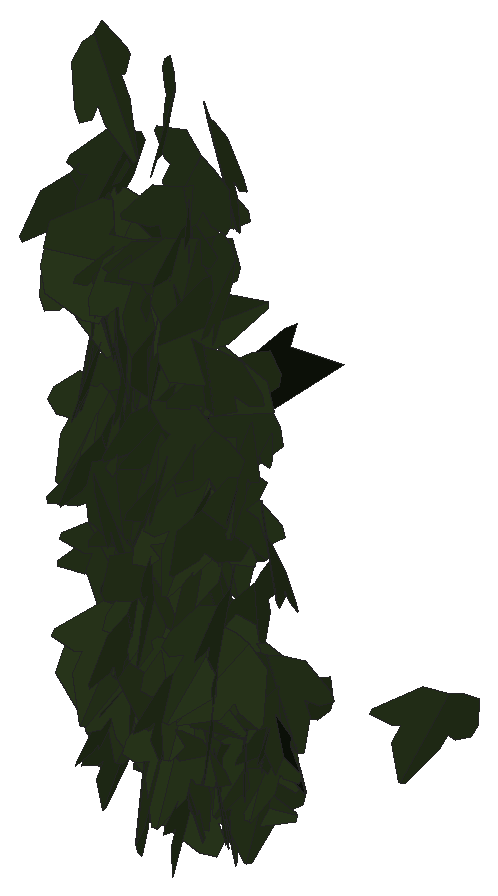
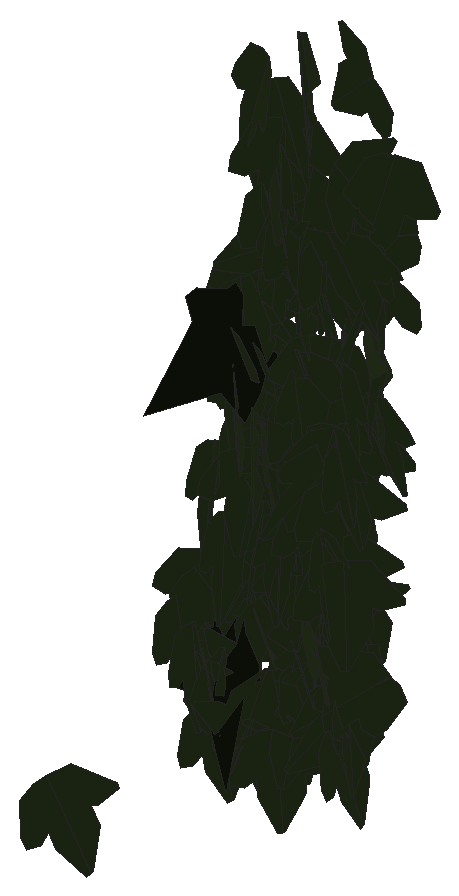
# SketchUp Ruby script. Lengths in inches.
U = 1.inch
M = Sketchup.active_model
def pt(a) = Geom::Point3d.new(a.map { |v| v * U })
def face(e, loops, mat)
  f = e.add_face(loops[0].map { |a| pt(a) })
  loops[1..].each { |l| e.add_face(l.map { |a| pt(a) }).erase! }
  f.material = f.back_material = mat if mat
  f
end
# faces: each face lists its corners as indices into pts; further lists are holes
def faces(e, pts, list, mat = nil) = list.each { |f| face(e, (f[0].is_a?(Array) ? f : [f]).map { |l| l.map { |i| pts[i] } }, mat) }
# xy, xz, yz: faces in a plane at the given z, y or x. An outline is a flat list of corners, or four numbers for a rectangle; further outlines are holes
def ring(l) = l.size == 4 ? [[l[0], l[1]], [l[2], l[1]], [l[2], l[3]], [l[0], l[3]]] : l.each_slice(2).to_a
def flat(e, list, mat, &to3) = list.each { |f| face(e, (f[0].is_a?(Array) ? f : [f]).map { |l| ring(l).map { |u, v| to3.(u, v) } }, mat) }
def xy(e, z, list, mat = nil) = flat(e, list, mat) { |x, y| [x, y, z] }
def xz(e, y, list, mat = nil) = flat(e, list, mat) { |x, z| [x, y, z] }
def yz(e, x, list, mat = nil) = flat(e, list, mat) { |y, z| [x, y, z] }
def lines(e, pts, list) = list.each { |a, b| e.add_line(pt(pts[a]), pt(pts[b])) }
# prism: a flat outline (further loops are holes) pulled along v
def prism(e, loops, v, mat = nil)
  f = face(e, loops, mat); d = Geom::Vector3d.new(v.map { |x| x * U })
  f.pushpull(f.normal.samedirection?(d) ? d.length : -d.length)
end
def box(e, o, s, mat = nil) = prism(e, [[o, [o[0] + s[0], o[1], o[2]], [o[0] + s[0], o[1] + s[1], o[2]], [o[0], o[1] + s[1], o[2]]]], [0, 0, s[2]], mat)
def at(x, y, z, deg = 0) = Geom::Transformation.translation(pt([x, y, z])) * Geom::Transformation.rotation(ORIGIN, Z_AXIS, deg.degrees)
def axes(o, x, y, z) = Geom::Transformation.new([*x, 0, *y, 0, *z, 0, *pt(o).to_a, 1])
def part(name) = M.definitions.add(name)
# library, detail: a bought-in or finely detailed component or shape, given as its bounding box
def library(name, o, s) = part(name).tap { |d| box(d.entities, o, s) }
def detail(e, o, s) = box(e.add_group.entities, o, s)
def put(e, d, t, mat = nil) = e.add_instance(d, t).tap { |i| i.material = mat if mat }
def group(e, t, mat = nil) = e.add_group.tap { |g| g.transformation = t; g.material = mat if mat }.entities
root = M.entities
M.materials.add("efeu1").color = [18, 25, 13]
M.materials.add("efeu2").color = [43, 57, 29]
c1 = part("ivyleaf_10")
p = [[0,0.5,-0.03],[-0.0625,2.02,-0.43],[-0.19,2.01,-0.46],[-0.54,1.05,-0.29],[-0.52,0.625,-0.18],[-0.83,0.76,-0.28],
  [-1.16,0.64,-0.33],[-1.15,0.33,-0.24],[-0.77,-0.39,0.02],[-0.3,-0.51,0.16],[0.04,-0.48,0.23],[-0.02,2.01,-0.4375],
  [-0.06,2.01,-0.43],[0.04,-0.49,0.23],[0.67,-0.49,0.14],[1.38,0.36,-0.2],[1.375,0.51,-0.24],[0.81,0.65,-0.19],
  [0.62,0.59,-0.15],[0.6,1.09,-0.28],[0.5,1.23,-0.31]]
faces(c1.entities,p,[[0,1,2,3,4,5,6,7,8,9,10],[11,12,0,13,14,15,16,17,18,19,20]],"efeu2")
c2 = part("ivyleaf_9")
p = [[1.54,2.16,1.25],[1.36,2.04,1.19],[-0.21,0.99,0.68],[-0.71,1.11,0.82],[-0.85,0.86,0.67],[-0.8,0.17,0.21],
  [-0.9,-0.01,0.1],[-0.67,-0.16,-0.02],[-0.08,-0.08,-0.05],[-0.03,-0.6,-0.4],[0.65,-0.88,-0.66],[0.83,-0.6,-0.49],
  [1.29,-0.42,-0.43],[1.8125,-0.07,-0.26],[1.21,0.44,0.15]]
faces(c2.entities,p,[[0,1,2,3,4,5,6,7,8,9,10,11,12,13,14]],"efeu1")
put(root,c1,axes([518.78,137.96,175.26],[-0.50751,-0.42588,0.04296],[-0.02362,-0.03868,-0.66237],[0.42739,-0.50785,0.01442]))
put(root,c1,axes([518.52,137.62,178.78],[-0.20052,0.24162,-0.60735],[0.13881,-0.60506,-0.28654],[-0.63874,-0.20734,0.1284]))
put(root,c1,axes([518.83,137.2,178.78],[0.29577,-0.57193,-0.26548],[-0.1065,0.24371,-0.64368],[0.62148,0.31395,0.01603]))
put(root,c1,axes([518.79,138.03,172.45],[0.05616,-0.64726,0.09818],[-0.00689,-0.09912,-0.64952],[0.65463,0.05449,-0.01526]))
put(root,c1,axes([518.35,137.83,173.59],[0.30727,0.26062,0.59411],[0.37634,0.46386,-0.39812],[-0.52845,0.48189,0.06192]))
put(root,c1,axes([518.9375,137.88,175.5625],[-0.4811,-0.41426,0.20769],[-0.13167,-0.16484,-0.6338],[0.44431,-0.49741,0.03707]))
put(root,c1,axes([518.85,137.18,177.88],[0.61337,-0.23963,-0.19798],[-0.18385,0.07347,-0.65852],[0.25064,0.64033,0.00147]))
put(root,c1,axes([518.9,137.61,173.06],[0.08241,-0.64908,-0.2337],[-0.04843,0.22934,-0.65404],[0.68817,0.09387,-0.01805]))
put(root,c1,axes([518.91,137.01,180.29],[0.45498,-0.40858,-0.34243],[-0.13516,0.34708,-0.59369],[0.51568,0.45145,0.14652]))
put(root,c1,axes([518.89,137.69,177.22],[-0.03414,-0.68527,0.01798],[0.00158,-0.01808,-0.68611],[0.6855,-0.03408,0.00247]))
put(root,c1,axes([519.05,137.875,177.49],[-0.61947,0.2017,0.17565],[-0.22489,-0.15298,-0.61749],[-0.14476,-0.62545,0.20768]))
put(root,c1,axes([518.98,137.75,176.5625],[-0.45983,-0.47966,0.11029],[-0.00425,-0.14707,-0.6573],[0.49216,-0.44942,0.09737]))
put(root,c1,axes([518.89,136.72,181.65],[-0.2605,-0.60194,-0.31695],[0.1428,0.28344,-0.65568],[0.66513,-0.29661,0.01664]))
put(root,c1,axes([518.54,137.18,180.16],[0.54281,0.04361,0.4176],[0.41722,0.02047,-0.54446],[-0.04706,0.68455,-0.01032]))
put(root,c1,axes([518.84,137.7,173.01],[-0.11754,-0.29919,-0.63473],[0.22771,0.59248,-0.32145],[0.66374,-0.25625,-0.00213]))
put(root,c1,axes([519.02,137.6,178.46],[0.49503,-0.39965,-0.24477],[-0.10959,0.24744,-0.62566],[0.45565,0.4937,0.11544]))
put(root,c1,axes([519.09,137.61,180.75],[0.74175,-0.00868,-0.18926],[-0.18925,0.00139,-0.7418],[0.00876,0.76552,-0.0008]))
put(root,c1,axes([519.07,137.45,181.92],[0.01775,-0.57438,0.40168],[0.06303,-0.39887,-0.57315],[0.69806,0.05062,0.04154]))
put(root,c1,axes([519.14,137.86,175.69],[0.069,-0.6441,-0.16655],[-0.01334,0.16607,-0.64777],[0.66515,0.07015,0.00428]))
put(root,c1,axes([519.03,137.28,179.55],[-0.31762,0.61017,-0.04957],[0.02418,-0.0433,-0.68789],[-0.6117,-0.31854,-0.00145]))
put(root,c1,axes([519.17,136.96,177.54],[-0.03487,-0.60794,-0.33331],[0.02309,0.33253,-0.60893],[0.69293,-0.04167,0.00352]))
put(root,c1,axes([519.17,137.33,174.41],[-0.28183,-0.5043,0.34703],[0.07091,-0.40636,-0.53293],[0.60804,-0.18635,0.223]))
put(root,c1,axes([519.15,137.09,176.83],[-0.26733,0.64252,0.07306],[-0.0214,0.07022,-0.69587],[-0.6463,-0.26809,-0.00718]))
put(root,c1,axes([519.09,137.85,173.8],[0.60477,0.26069,0.04446],[-0.00299,0.1177,-0.64948],[-0.26443,0.59487,0.10902]))
put(root,c1,axes([519.4,137.81,173.41],[-0.42158,-0.42863,0.25873],[-0.13762,-0.226,-0.59865],[0.48138,-0.44,0.05544]))
put(root,c1,axes([519.14,137.64,177.5],[0.35138,0.5763,-0.05904],[-0.03168,-0.04983,-0.67497],[-0.57845,0.3528,0.00111]))
put(root,c1,axes([519.11,137.5,173.59],[0.2572,0.60786,0.12352],[0.04796,0.11383,-0.66003],[-0.61842,0.26163,0.00018]))
put(root,c1,axes([519.13,137.91,174.2],[0.62156,0.19311,0.12015],[0.0362,0.26119,-0.60707],[-0.22454,0.57667,0.23473]))
put(root,c1,axes([519.35,137.0625,177.08],[-0.47387,-0.52713,-0.06108],[0.03954,0.04658,-0.70881],[0.52918,-0.47551,-0.00173]))
put(root,c1,axes([519.33,137.86,176.14],[-0.34525,-0.56999,-0.08475],[0.05101,0.06818,-0.66635],[0.574,-0.3489,0.00825]))
put(root,c1,axes([519.13,137.98,174.04],[0.27093,-0.50543,0.32939],[0.23241,-0.24577,-0.56828],[0.55673,0.34857,0.07694]))
put(root,c1,axes([519.375,137.71,177.18],[-0.35934,-0.58029,0.05926],[0.01993,-0.08178,-0.67992],[0.58297,-0.35489,0.05977]))
put(root,c1,axes([519.32,137.96,174.34],[0.21358,-0.61791,0.11175],[0.0144,-0.11319,-0.65338],[0.62777,0.21282,-0.02304]))
put(root,c1,axes([519.34,137.67,178.02],[-0.68151,-0.03436,-0.08463],[0.08909,-0.1094,-0.67297],[0.02016,-0.67798,0.11288]))
put(root,c1,axes([519.5,137.37,180.44],[-0.17025,-0.65447,0.15746],[-0.02726,-0.15558,-0.67614],[0.67259,-0.17197,0.01245]))
put(root,c1,axes([519.43,137.64,174.66],[0.32192,-0.50495,-0.29194],[-0.00944,0.3289,-0.57929],[0.58319,0.28406,0.15177]))
put(root,c1,axes([518.96,136.54,180.61],[0.06451,0.0972,0.73673],[0.50799,0.53396,-0.11493],[-0.54237,0.51168,-0.02002]))
put(root,c1,axes([519.26,137.77,176.9375],[-0.20609,-0.40817,-0.49563],[0.34267,0.37028,-0.44743],[0.54298,-0.3886,0.09425]))
put(root,c1,axes([518.98,137.09,183.49],[0.44515,-0.1185,0.58486],[0.58062,-0.08248,-0.45863],[0.13779,0.73035,0.0431]))
put(root,c1,axes([519.49,137.5,178.68],[-0.63399,-0.26382,-0.0744],[0.11198,-0.07817,-0.67707],[0.25019,-0.63354,0.11452]))
put(root,c1,axes([519.54,138.03,173.72],[0.39481,-0.52936,-0.00765],[-0.01138,0.00105,-0.66032],[0.52929,0.39488,-0.00849]))
put(root,c1,axes([519.61,138.05,172.9375],[-0.63628,-0.16446,-0.02013],[0.01648,0.0167,-0.65708],[0.16487,-0.63638,-0.01204]))
put(root,c1,axes([519.59,136.97,174.83],[0.05137,-0.61998,-0.28428],[0.0371,0.2872,-0.61965],[0.68104,0.03112,0.0552]))
put(root,c1,axes([519.86,136.51,179.14],[-0.00724,-0.03018,-0.71368],[-0.2842,0.65492,-0.02481],[0.65535,0.28368,-0.01865]))
put(root,c1,axes([519.49,137.79,174.9],[-0.23865,0.48237,-0.40974],[0.11705,-0.39671,-0.53521],[-0.62199,-0.25974,0.0565]))
put(root,c1,axes([519.48,137.93,175.87],[0.64812,-0.04807,0.13555],[0.13545,-0.00625,-0.64989],[0.04834,0.66211,0.0037]))
put(root,c1,axes([519.92,136.9375,171.9],[0.33145,-0.29587,0.60951],[-0.46645,0.39248,0.44417],[-0.4914,-0.57212,-0.01051]))
put(root,c1,axes([519.6875,137.63,178.5],[0.673,-0.10199,-0.12283],[-0.11417,0.06452,-0.67913],[0.1116,0.68107,0.04594]))
put(root,c1,axes([519.79,138.32,172.19],[-0.49737,-0.39098,0.07189],[-0.03428,-0.07252,-0.63165],[0.39605,-0.49728,0.0356]))
put(root,c1,axes([519.8,137.78,174.98],[-0.11691,-0.43206,0.49455],[-0.03689,-0.49722,-0.44311],[0.65567,-0.10502,0.06325]))
put(root,c1,axes([519.79,137.41,178.07],[-0.17726,-0.63315,-0.1793],[0.05859,0.16977,-0.65742],[0.65544,-0.18641,0.01028]))
put(root,c1,axes([519.93,137.67,177.7],[-0.08079,-0.68139,0.05158],[-0.00728,-0.05107,-0.68616],[0.6833,-0.08111,-0.00121]))
put(root,c1,axes([520.02,138.01,175.63],[-0.599,0.22774,0.16973],[-0.1782,0.00715,-0.63849],[-0.22117,-0.62254,0.05476]))
put(root,c1,axes([519.82,137.47,175.06],[0.44559,0.48295,-0.15155],[-0.09681,-0.11686,-0.65706],[-0.49683,0.45592,-0.00788]))
put(root,c1,axes([519.84,137.2,179.7],[0.48658,-0.49968,0.04922],[0.06635,-0.00395,-0.69602],[0.4977,0.48904,0.04467]))
put(root,c1,axes([519.98,137.22,180.32],[-0.58741,0.36009,0.06976],[-0.08074,0.00153,-0.6878],[-0.35779,-0.59154,0.04068]))
put(root,c1,axes([519.84,136.99,180.51],[0.40347,0.56481,-0.00031],[-0.00021,-0.00023,-0.69412],[-0.56481,0.40347,0.00003]))
put(root,c1,axes([519.9,137.87,176.5],[0.66192,0.08591,-0.01452],[-0.01485,0.00162,-0.66746],[-0.08586,0.66207,0.00352]))
put(root,c1,axes([520.09,137.375,180.7],[-0.23086,-0.65579,0.11632],[-0.02119,-0.11582,-0.695],[0.66569,-0.23111,0.01822]))
put(root,c1,axes([520.04,137.05,177.5],[0.47001,-0.48559,-0.08372],[-0.05759,0.06076,-0.6758],[0.48938,0.47352,0.00087]))
put(root,c1,axes([520.06,137.44,176.99],[0.05832,-0.66018,0.16754],[0.02386,-0.16606,-0.66269],[0.68069,0.06239,0.00888]))
put(root,c1,axes([520.125,137.13,180.77],[-0.44256,-0.55487,-0.0039],[0.01412,-0.00627,-0.7096],[0.55471,-0.44254,0.01495]))
put(root,c1,axes([519.78,137.55,179.56],[0.14247,-0.37329,0.56187],[0.3909,-0.42233,-0.3797],[0.54976,0.39703,0.12437]))
put(root,c1,axes([519.96,137.33,175.64],[-0.05415,0.4966,-0.4529],[-0.00189,-0.45448,-0.49811],[-0.67211,-0.03873,0.03789]))
put(root,c1,axes([520.11,136.57,179.65],[0.06087,0.01636,-0.71351],[-0.0013,0.7161,0.01631],[0.7137,-0.00009,0.06089]))
put(root,c1,axes([519.75,137.8,172.71],[-0.31903,0.36771,-0.58844],[0.39695,-0.4345,-0.48673],[-0.56913,-0.50917,-0.00962]))
put(root,c1,axes([520.29,137.79,174.11],[-0.41686,-0.36812,0.37167],[-0.10586,-0.40606,-0.5209],[0.51229,-0.38345,0.1948]))
put(root,c1,axes([520.01,136.99,175.88],[-0.60742,-0.2101,-0.29813],[0.29068,0.07091,-0.64222],[0.22028,-0.67291,0.02541]))
put(root,c1,axes([520.17,137.1875,181.27],[-0.67682,0.14275,-0.03308],[0.03295,-0.00407,-0.6917],[-0.14278,-0.67761,-0.00281]))
put(root,c1,axes([520.25,138.43,172.48],[0.51404,0.35315,0.14437],[-0.14249,-0.047,0.62232],[0.35391,-0.53185,0.04086]))
put(root,c1,axes([519.92,137.56,176.06],[0.65833,-0.03637,0.27245],[0.2731,0.00655,-0.65904],[0.0311,0.71245,0.01997]))
put(root,c1,axes([520.33,136.95,183.38],[0.32342,-0.54059,-0.35961],[-0.12631,0.3417,-0.62725],[0.63687,0.34229,0.05822]))
put(root,c1,axes([520.33,137.47,172.28],[0.26151,-0.60075,0.07958],[0.05926,-0.06091,-0.65452],[0.60309,0.26648,0.02981]))
put(root,c1,axes([520.41,137.34,181.17],[0.19216,-0.68006,-0.0418],[0.00736,0.0455,-0.70642],[0.6813,0.19132,0.01943]))
put(root,c1,axes([520.49,137.54,176.87],[0.21543,-0.62278,-0.24174],[-0.07636,0.22938,-0.65898],[0.66367,0.22854,0.00265]))
put(root,c1,axes([520.44,137.57,176.96],[0.6085,-0.25398,-0.12296],[-0.10476,0.06807,-0.659],[0.26202,0.61705,0.02209]))
put(root,c1,axes([520.3125,137.39,176.49],[0.42107,0.52899,-0.03109],[-0.02119,-0.02287,-0.67611],[-0.52948,0.4216,0.00233]))
put(root,c1,axes([520.32,137.43,181.74],[0.4454,-0.53247,0.01746],[0.13902,0.09419,-0.67381],[0.5143,0.43568,0.16701]))
put(root,c1,axes([520.49,136.92,174.26],[0.12649,-0.66773,-0.03536],[-0.00105,0.03578,-0.67958],[0.66866,0.12637,0.00562]))
put(root,c1,axes([520.375,137.04,173.25],[0.64209,-0.03248,-0.01708],[-0.01715,-0.0008,-0.64291],[0.03245,0.64232,-0.00167]))
put(root,c1,axes([520.61,137.75,177.13],[0.16971,-0.47142,-0.46343],[-0.14429,0.44051,-0.50094],[0.64512,0.22254,0.00987]))
put(root,c1,axes([520.47,137.03,173.2],[-0.65731,0.11246,-0.06956],[0.06789,-0.01563,-0.66684],[-0.11347,-0.66079,0.00394]))
put(root,c1,axes([519.94,137.84,171.96],[0.06502,-0.0032,0.76231],[0.61484,0.45253,-0.05054],[-0.45067,0.6169,0.04103]))
put(root,c1,axes([520.82,137,182.43],[-0.60661,0.13389,0.36427],[-0.38137,-0.08032,-0.60557],[-0.07196,-0.70301,0.13856]))
put(root,c1,axes([520.6,137.15,180.92],[-0.36487,-0.59555,0.12564],[-0.01833,-0.13567,-0.69631],[0.60838,-0.36126,0.05437]))
put(root,c1,axes([520.45,138.02,172.36],[-0.27377,0.57291,-0.11289],[0.03609,-0.10785,-0.63481],[-0.58281,-0.27579,0.01372]))
put(root,c1,axes([520.625,137.04,181.85],[-0.57931,-0.38426,-0.03726],[0.03003,0.02214,-0.69517],[0.3849,-0.58008,-0.00184]))
put(root,c1,axes([520.53,137.32,174.41],[0.33238,0.55106,-0.23253],[-0.11685,-0.20107,-0.64353],[-0.58658,0.3523,-0.00356]))
put(root,c1,axes([520.6,137.83,176.51],[-0.57337,-0.35064,-0.07902],[0.09846,-0.01014,-0.66944],[0.34569,-0.5787,0.05961]))
put(root,c1,axes([520.63,137.32,176.94],[0.33458,0.53734,-0.24738],[-0.20684,-0.15999,-0.62729],[-0.55421,0.38411,0.08478]))
put(root,c1,axes([520.51,137.45,176.66],[0.73504,0.06993,-0.02019],[-0.02085,0.00595,-0.73832],[-0.06974,0.73529,0.00789]))
put(root,c1,axes([520.18,136.86,174.31],[-0.39041,-0.02275,-0.61158],[0.6102,0.04119,-0.39106],[0.04695,-0.7244,-0.00303]))
put(root,c1,axes([520.99,136.98,178.2],[-0.53464,-0.07883,0.42758],[-0.40213,-0.16803,-0.5338],[0.16532,-0.66365,0.08436]))
put(root,c1,axes([520.55,137.45,175.67],[0.09346,-0.63292,-0.20987],[0.17139,0.22761,-0.61007],[0.6444,0.03126,0.1927]))
put(root,c2,axes([520.96,138.13,173.54],[0.44123,0.08611,-0.61161],[-0.60729,-0.07656,-0.4489],[-0.11261,0.75026,0.02439]))
put(root,c1,axes([520.92,137.4,172.63],[-0.30828,0.50594,0.23881],[-0.22198,0.13967,-0.58246],[-0.51355,-0.36409,0.10841]))
put(root,c1,axes([521,137.89,173.125],[-0.28734,0.54467,0.20836],[-0.28017,0.07478,-0.58186],[-0.51145,-0.34697,0.20167]))
put(root,c1,axes([521,138.25,172.23],[-0.29437,-0.55661,0.109],[-0.01477,-0.11524,-0.62837],[0.56699,-0.29199,0.04022]))
put(root,c1,axes([520.65,137.625,174.03],[0.36415,-0.37085,0.47842],[0.34852,-0.32804,-0.51956],[0.49492,0.50387,0.01387]))
put(root,c1,axes([520.98,137.27,175.03],[0.29803,0.47466,-0.40116],[-0.23038,-0.32883,-0.56022],[-0.5772,0.37633,0.01647]))
put(root,c1,axes([520.95,138.29,173],[-0.14969,-0.41914,0.45869],[0.0586,-0.47923,-0.41879],[0.61858,-0.05603,0.15067]))
put(root,c1,axes([521.09,137.68,177.79],[0.25676,-0.47376,-0.42549],[-0.17677,0.38772,-0.53837],[0.61176,0.31088,0.02302]))
put(root,c1,axes([520.86,136.625,179.93],[0.07063,-0.07207,0.71549],[0.01011,0.71896,0.07142],[-0.71904,0.00303,0.07129]))
put(root,c1,axes([521.01,137.97,175.35],[-0.01593,-0.63857,-0.21042],[0.02734,0.20969,-0.63842],[0.67179,-0.02367,0.02099]))
put(root,c1,axes([520.51,138.2,173.15],[0.35026,0.03309,0.54247],[0.52029,0.16609,-0.34607],[-0.15706,0.62399,0.06335]))
put(root,c1,axes([521.1,136.9375,179.52],[-0.68678,-0.01609,0.06992],[-0.0698,-0.00574,-0.68696],[0.01659,-0.69031,0.00408]))
put(root,c1,axes([520.98,137.5,178.1],[-0.17165,-0.63889,-0.1522],[0.11655,0.12518,-0.65693],[0.64635,-0.19224,0.07804]))
put(root,c1,axes([521.01,137.21,182.92],[-0.549,0.43286,-0.04095],[0.01294,-0.04966,-0.69843],[-0.4346,-0.54828,0.03093]))
put(root,c2,axes([521.05,137.66,178.74],[-0.12564,0.24535,-0.72939],[-0.30089,0.66455,0.27537],[0.70828,0.32583,-0.0124]))
put(root,c1,axes([521.11,137.45,179.1],[-0.28924,-0.63808,0.02152],[0.01376,-0.02984,-0.70014],[0.6383,-0.2885,0.02484]))
put(root,c1,axes([521.26,137.18,174.76],[0.58654,0.00229,-0.36569],[-0.36561,0.01815,-0.58631],[0.00766,0.69096,0.01661]))
put(root,c1,axes([521.09,138.37,173.42],[0.33907,-0.54519,-0.06077],[-0.00404,0.06896,-0.64119],[0.54855,0.3375,0.03285]))
put(root,c1,axes([521.04,138.25,173.03],[0.62363,-0.12873,-0.0014],[-0.00074,0.00332,-0.63677],[0.12874,0.62362,0.0031]))
put(root,c1,axes([521.67,137.22,178.81],[-0.21812,-0.00911,0.66246],[-0.62675,-0.22322,-0.20944],[0.21474,-0.66076,0.06162]))
put(root,c1,axes([521.43,137.9375,174.28],[-0.37481,-0.34136,0.4119],[-0.25717,-0.32603,-0.50422],[0.4691,-0.45149,0.05268]))
put(root,c1,axes([521.32,136.92,181],[0.44705,-0.50313,-0.2244],[-0.15411,0.16323,-0.67302],[0.5289,0.47283,-0.00643]))
put(root,c1,axes([521.49,137.82,176.33],[-0.49099,0.33264,0.32838],[-0.28329,0.16705,-0.59279],[-0.37179,-0.56657,0.01801]))
put(root,c1,axes([521.34,136.93,175.82],[0.22122,-0.60992,-0.14111],[-0.01937,0.14293,-0.64811],[0.62573,0.22005,0.02983]))
put(root,c1,axes([521.37,138.26,173.43],[-0.05064,-0.64206,-0.09498],[0.00379,0.09497,-0.64404],[0.64904,-0.05065,-0.00365]))
put(root,c1,axes([521.49,141.5,172.19],[-0.3046,-0.53097,0.24391],[-0.13516,-0.20357,-0.61196],[0.56847,-0.33291,-0.01481]))
put(root,c1,axes([521.27,136.77,177.22],[-0.24119,-0.49257,-0.46586],[0.19601,0.42269,-0.5484],[0.64902,-0.3107,-0.00751]))
put(root,c1,axes([521.35,137.57,178.5],[0.59748,-0.32328,0.03595],[0.0357,-0.00956,-0.67927],[0.32331,0.59848,0.00857]))
put(root,c1,axes([521.28,137.24,178.23],[0.60736,-0.27379,0.16454],[0.16847,-0.02577,-0.66474],[0.27139,0.62872,0.04441]))
put(root,c1,axes([521.62,138.22,173.83],[-0.16253,-0.626,0.08958],[-0.01525,-0.08858,-0.64671],[0.63219,-0.16307,0.00743]))
put(root,c1,axes([521.55,137.82,174.4],[-0.64518,-0.08263,-0.08152],[0.08405,-0.01502,-0.64995],[0.08006,-0.65013,0.02537]))
